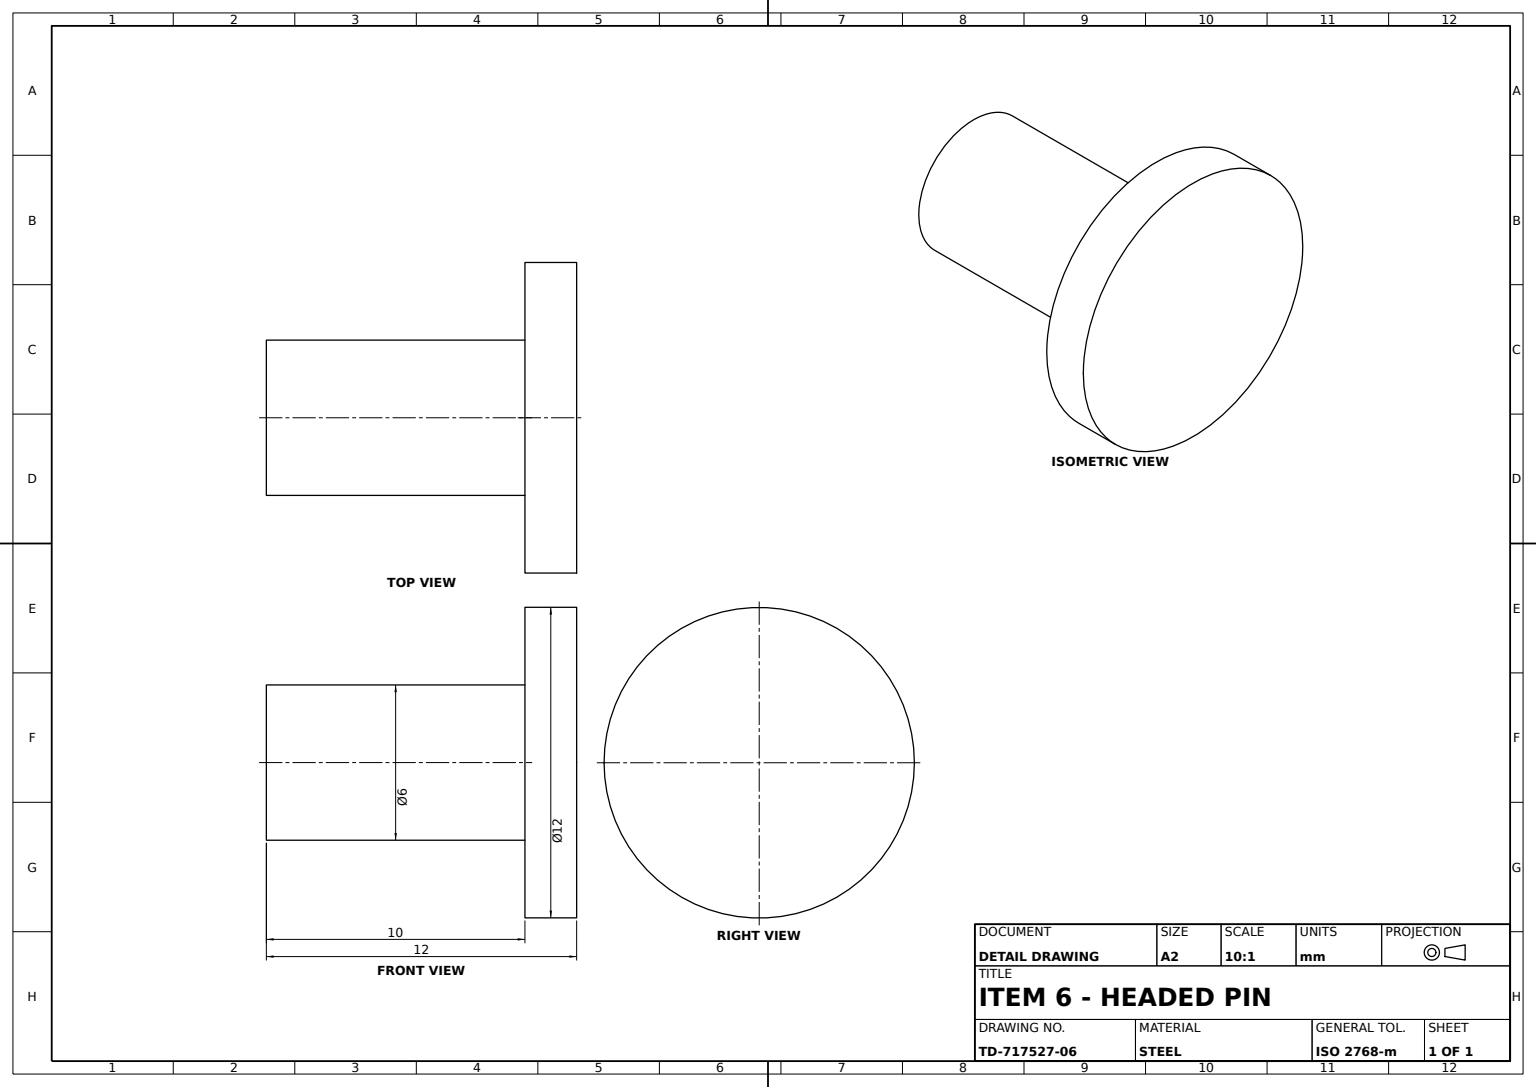
ISO-10303-21;
HEADER;
FILE_DESCRIPTION((''),'2;1');
FILE_NAME('','',(''),(''),'','','');
FILE_SCHEMA(('AUTOMOTIVE_DESIGN'));
ENDSEC;
DATA;
#1=APPLICATION_CONTEXT('');
#2=PRODUCT_CONTEXT('',#1,'mechanical');
#3=PRODUCT('','','',(#2));
#4=PRODUCT_DEFINITION_FORMATION('','',#3);
#5=PRODUCT_DEFINITION_CONTEXT('',#1,'design');
#6=PRODUCT_DEFINITION('','',#4,#5);
#7=PRODUCT_DEFINITION_SHAPE('','',#6);
#8=(LENGTH_UNIT()NAMED_UNIT(*)SI_UNIT(.MILLI.,.METRE.));
#9=(NAMED_UNIT(*)PLANE_ANGLE_UNIT()SI_UNIT($,.RADIAN.));
#10=(NAMED_UNIT(*)SI_UNIT($,.STERADIAN.)SOLID_ANGLE_UNIT());
#11=UNCERTAINTY_MEASURE_WITH_UNIT(LENGTH_MEASURE(1.E-05),#8,'distance_accuracy_value','');
#12=(GEOMETRIC_REPRESENTATION_CONTEXT(3)GLOBAL_UNCERTAINTY_ASSIGNED_CONTEXT((#11))GLOBAL_UNIT_ASSIGNED_CONTEXT((#8,#9,#10))REPRESENTATION_CONTEXT('',''));
#13=CARTESIAN_POINT('',(0.,0.,3.));
#14=VERTEX_POINT('',#13);
#15=CARTESIAN_POINT('',(0.,0.,-3.));
#16=VERTEX_POINT('',#15);
#17=CARTESIAN_POINT('',(0.,0.,0.));
#18=DIRECTION('',(0.,1.,0.));
#19=DIRECTION('',(0.,0.,1.));
#20=AXIS2_PLACEMENT_3D('',#17,#18,#19);
#21=CIRCLE('',#20,3.);
#22=EDGE_CURVE('',#14,#16,#21,.T.);
#23=ORIENTED_EDGE('',*,*,#22,.F.);
#24=EDGE_CURVE('',#16,#14,#21,.T.);
#25=ORIENTED_EDGE('',*,*,#24,.F.);
#26=EDGE_LOOP('',(#23,#25));
#27=FACE_OUTER_BOUND('',#26,.T.);
#28=PLANE('',#20);
#29=ADVANCED_FACE('',(#27),#28,.F.);
#30=CARTESIAN_POINT('',(0.,12.,-6.));
#31=VERTEX_POINT('',#30);
#32=CARTESIAN_POINT('',(0.,12.,6.));
#33=VERTEX_POINT('',#32);
#34=CARTESIAN_POINT('',(0.,12.,0.));
#35=AXIS2_PLACEMENT_3D('',#34,#18,#19);
#36=CIRCLE('',#35,6.);
#37=EDGE_CURVE('',#31,#33,#36,.T.);
#38=ORIENTED_EDGE('',*,*,#37,.T.);
#39=EDGE_CURVE('',#33,#31,#36,.T.);
#40=ORIENTED_EDGE('',*,*,#39,.T.);
#41=EDGE_LOOP('',(#38,#40));
#42=FACE_OUTER_BOUND('',#41,.T.);
#43=PLANE('',#35);
#44=ADVANCED_FACE('',(#42),#43,.T.);
#45=CARTESIAN_POINT('',(0.,10.,-3.));
#46=VERTEX_POINT('',#45);
#47=CARTESIAN_POINT('',(0.,10.,3.));
#48=VERTEX_POINT('',#47);
#49=CARTESIAN_POINT('',(0.,10.,0.));
#50=AXIS2_PLACEMENT_3D('',#49,#18,#19);
#51=CIRCLE('',#50,3.);
#52=EDGE_CURVE('',#46,#48,#51,.T.);
#53=ORIENTED_EDGE('',*,*,#52,.T.);
#54=EDGE_CURVE('',#48,#46,#51,.T.);
#55=ORIENTED_EDGE('',*,*,#54,.T.);
#56=EDGE_LOOP('',(#53,#55));
#57=FACE_BOUND('',#56,.T.);
#58=CARTESIAN_POINT('',(0.,10.,-6.));
#59=VERTEX_POINT('',#58);
#60=CARTESIAN_POINT('',(0.,10.,6.));
#61=VERTEX_POINT('',#60);
#62=CIRCLE('',#50,6.);
#63=EDGE_CURVE('',#59,#61,#62,.T.);
#64=ORIENTED_EDGE('',*,*,#63,.F.);
#65=EDGE_CURVE('',#61,#59,#62,.T.);
#66=ORIENTED_EDGE('',*,*,#65,.F.);
#67=EDGE_LOOP('',(#64,#66));
#68=FACE_OUTER_BOUND('',#67,.T.);
#69=PLANE('',#50);
#70=ADVANCED_FACE('',(#57,#68),#69,.F.);
#71=ORIENTED_EDGE('',*,*,#63,.T.);
#72=DIRECTION('',(0.,-1.,0.));
#73=VECTOR('',#72,1000.);
#74=LINE('',#32,#73);
#75=EDGE_CURVE('',#33,#61,#74,.T.);
#76=ORIENTED_EDGE('',*,*,#75,.F.);
#77=ORIENTED_EDGE('',*,*,#37,.F.);
#78=LINE('',#30,#73);
#79=EDGE_CURVE('',#31,#59,#78,.T.);
#80=ORIENTED_EDGE('',*,*,#79,.T.);
#81=EDGE_LOOP('',(#71,#76,#77,#80));
#82=FACE_OUTER_BOUND('',#81,.T.);
#83=DIRECTION('',(0.,0.,-1.));
#84=AXIS2_PLACEMENT_3D('',#34,#72,#83);
#85=CYLINDRICAL_SURFACE('',#84,6.);
#86=ADVANCED_FACE('',(#82),#85,.T.);
#87=ORIENTED_EDGE('',*,*,#22,.T.);
#88=LINE('',#45,#73);
#89=EDGE_CURVE('',#46,#16,#88,.T.);
#90=ORIENTED_EDGE('',*,*,#89,.F.);
#91=ORIENTED_EDGE('',*,*,#54,.F.);
#92=LINE('',#47,#73);
#93=EDGE_CURVE('',#48,#14,#92,.T.);
#94=ORIENTED_EDGE('',*,*,#93,.T.);
#95=EDGE_LOOP('',(#87,#90,#91,#94));
#96=FACE_OUTER_BOUND('',#95,.T.);
#97=AXIS2_PLACEMENT_3D('',#49,#72,#83);
#98=CYLINDRICAL_SURFACE('',#97,3.);
#99=ADVANCED_FACE('',(#96),#98,.T.);
#100=ORIENTED_EDGE('',*,*,#75,.T.);
#101=ORIENTED_EDGE('',*,*,#65,.T.);
#102=ORIENTED_EDGE('',*,*,#79,.F.);
#103=ORIENTED_EDGE('',*,*,#39,.F.);
#104=EDGE_LOOP('',(#100,#101,#102,#103));
#105=FACE_OUTER_BOUND('',#104,.T.);
#106=ADVANCED_FACE('',(#105),#85,.T.);
#107=ORIENTED_EDGE('',*,*,#24,.T.);
#108=ORIENTED_EDGE('',*,*,#93,.F.);
#109=ORIENTED_EDGE('',*,*,#52,.F.);
#110=ORIENTED_EDGE('',*,*,#89,.T.);
#111=EDGE_LOOP('',(#107,#108,#109,#110));
#112=FACE_OUTER_BOUND('',#111,.T.);
#113=ADVANCED_FACE('',(#112),#98,.T.);
#114=CLOSED_SHELL('',(#29,#44,#70,#86,#99,#106,#113));
#115=MANIFOLD_SOLID_BREP('',#114);
#116=ADVANCED_BREP_SHAPE_REPRESENTATION('',(#115),#12);
#117=SHAPE_DEFINITION_REPRESENTATION(#7,#116);
ENDSEC;
END-ISO-10303-21;
